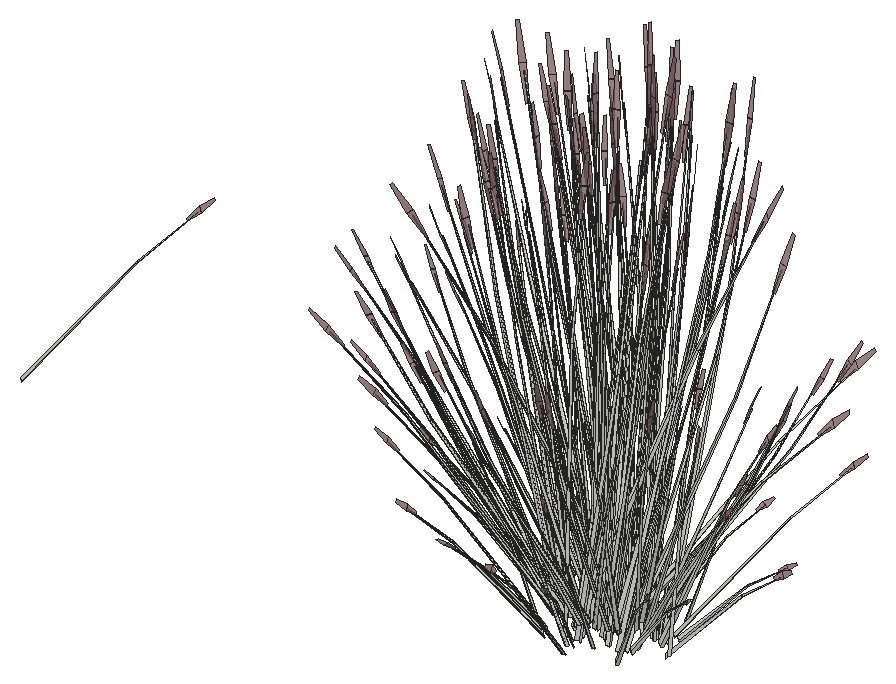
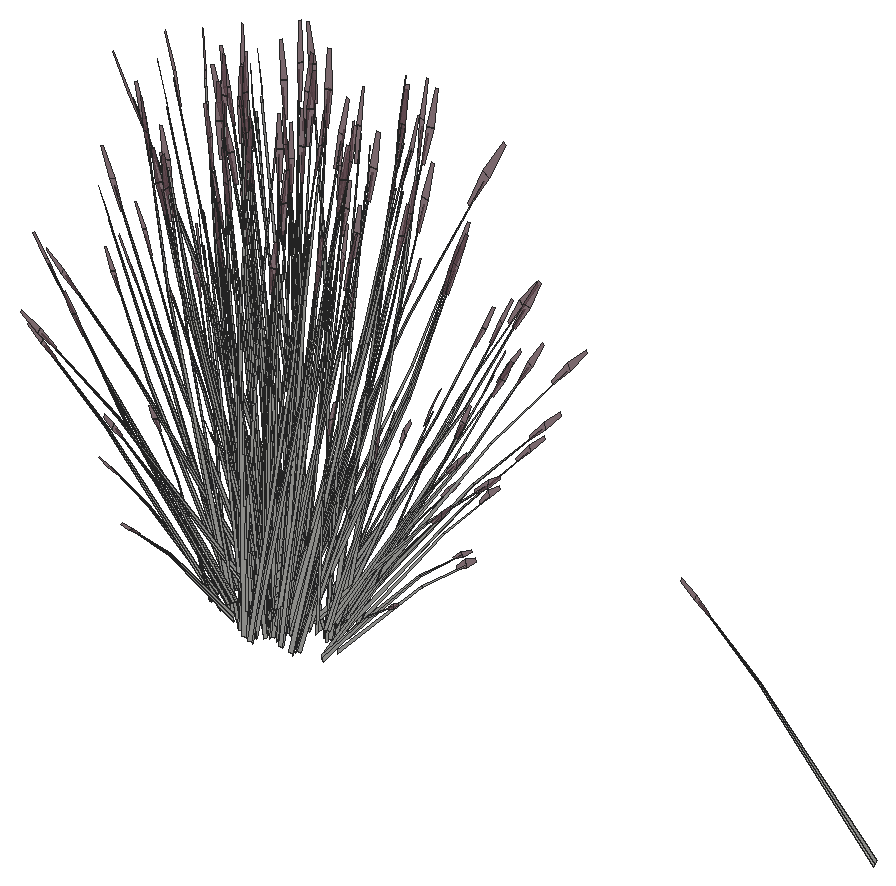
# SketchUp Ruby script. Lengths in millimetres.
U = 1.mm
M = Sketchup.active_model
def pt(a) = Geom::Point3d.new(a.map { |v| v * U })
def face(e, loops, mat)
  f = e.add_face(loops[0].map { |a| pt(a) })
  loops[1..].each { |l| e.add_face(l.map { |a| pt(a) }).erase! }
  f.material = f.back_material = mat if mat
  f
end
# faces: each face lists its corners as indices into pts; further lists are holes
def faces(e, pts, list, mat = nil) = list.each { |f| face(e, (f[0].is_a?(Array) ? f : [f]).map { |l| l.map { |i| pts[i] } }, mat) }
# xy, xz, yz: faces in a plane at the given z, y or x. An outline is a flat list of corners, or four numbers for a rectangle; further outlines are holes
def ring(l) = l.size == 4 ? [[l[0], l[1]], [l[2], l[1]], [l[2], l[3]], [l[0], l[3]]] : l.each_slice(2).to_a
def flat(e, list, mat, &to3) = list.each { |f| face(e, (f[0].is_a?(Array) ? f : [f]).map { |l| ring(l).map { |u, v| to3.(u, v) } }, mat) }
def xy(e, z, list, mat = nil) = flat(e, list, mat) { |x, y| [x, y, z] }
def xz(e, y, list, mat = nil) = flat(e, list, mat) { |x, z| [x, y, z] }
def yz(e, x, list, mat = nil) = flat(e, list, mat) { |y, z| [x, y, z] }
def lines(e, pts, list) = list.each { |a, b| e.add_line(pt(pts[a]), pt(pts[b])) }
# prism: a flat outline (further loops are holes) pulled along v
def prism(e, loops, v, mat = nil)
  f = face(e, loops, mat); d = Geom::Vector3d.new(v.map { |x| x * U })
  f.pushpull(f.normal.samedirection?(d) ? d.length : -d.length)
end
def box(e, o, s, mat = nil) = prism(e, [[o, [o[0] + s[0], o[1], o[2]], [o[0] + s[0], o[1] + s[1], o[2]], [o[0], o[1] + s[1], o[2]]]], [0, 0, s[2]], mat)
def at(x, y, z, deg = 0) = Geom::Transformation.translation(pt([x, y, z])) * Geom::Transformation.rotation(ORIGIN, Z_AXIS, deg.degrees)
def axes(o, x, y, z) = Geom::Transformation.new([*x, 0, *y, 0, *z, 0, *pt(o).to_a, 1])
def part(name) = M.definitions.add(name)
# library, detail: a bought-in or finely detailed component or shape, given as its bounding box
def library(name, o, s) = part(name).tap { |d| box(d.entities, o, s) }
def detail(e, o, s) = box(e.add_group.entities, o, s)
def put(e, d, t, mat = nil) = e.add_instance(d, t).tap { |i| i.material = mat if mat }
def group(e, t, mat = nil) = e.add_group.tap { |g| g.transformation = t; g.material = mat if mat }.entities
root = M.entities
M.materials.add("LightPink_Translucent").color = [144, 107, 117]
M.materials["LightPink_Translucent"].alpha = 0.8
c1 = part("blade")
p = [[54.7,5.3,558.8],[0,4.4,0],[2.3,11.5,0],[55.5,7.8,558.8],[58.2,7.8,558.8],[9.8,11.5,0],
  [62.9,5.7,838.2],[63,6,838.2],[63.4,6,838.2]]
faces(c1.entities,p,[[0,1,2,3],[4,5,2,3],[6,0,3,7],[7,3,4,8]])
c2 = part("seeds")
p = [[7.6,-2.7,35.1],[-0.2,-0.6,40.4],[-0.2,-0.8,0.9],[3.5,-1.8,-1.7],[7.5,-0.8,76.3],[3.7,0.2,78.9]]
faces(c2.entities,p,[[0,1,2,3],[1,0,4,5]],"LightPink_Translucent")
c3 = part("blade with seeds")
put(c3.entities,c1,at(0,0,0))
put(c3.entities,c2,axes([60.9,6.5,787.2],[1.5799,-0.05474,1.17369],[-0.12525,1.92788,0.29478],[-0.07173,-0.02425,1.56792]))
put(root,c3,axes([14344.8,4419.7,8470.3],[-0.29514,-0.25472,1.43002],[0.38401,-0.84262,-0.30754],[0.59714,0.11414,0.61141]))
put(root,c3,axes([16061.4,4330.2,8503],[0.50831,-0.02346,1.71376],[-0.33721,1.01661,0.13857],[-0.72439,-0.06288,0.73262]))
put(root,c3,axes([16066.8,4375.7,8503],[0.42521,-0.21906,1.71376],[0.35798,1.01226,0.13857],[-0.66754,0.22878,0.73262]))
put(root,c3,axes([16033.2,4419.5,8470.3],[0.42589,0.08502,1.43002],[0.2745,0.86839,-0.30754],[-0.57851,0.16255,0.61141]))
put(root,c3,axes([16128.9,4348.8,8489.4],[0.34834,-0.14982,1.77064],[0.12012,1.04605,0.13857],[-0.75452,0.1388,0.63284]))
put(root,c3,axes([16100.1,4306.2,8531],[-1.22504,-0.02494,-0.71045],[0.08228,-1.05005,0.08574],[-0.51899,-0.11081,1.00501]))
put(root,c3,axes([16075,4312.7,8470.3],[0.23927,0.28834,1.43002],[-0.55135,0.78376,-0.30754],[-0.56612,-0.18733,0.61141]))
put(root,c3,axes([16050.1,4352.4,8519.5],[-1.01846,-0.28891,-0.35414],[0.29705,-0.84289,0.4572],[-0.41005,0.07729,0.87481]))
put(root,c3,axes([16085.8,4288.8,8503],[0.45521,0.17844,1.71376],[-0.94204,0.74856,0.13857],[-0.58713,-0.33769,0.73262]))
put(root,c3,axes([16067.8,4363.3,8523.4],[-0.332,0.94205,-0.51099],[-1.13828,-0.3229,-0.3958],[-0.45829,0.08638,0.97773]))
put(root,c3,axes([16089.7,4311.6,8523.4],[-0.88986,0.68603,-0.51099],[-0.77932,-0.72471,-0.3958],[-0.45212,-0.10438,0.97773]))
put(root,c3,axes([16053.3,4361.8,8442.4],[0.03108,0.16322,1.76342],[-0.62654,0.85237,-0.26939],[-0.44504,-0.04296,0.30037]))
put(root,c3,axes([16010.6,4465.7,8474.7],[0.51072,-0.46938,1.1486],[0.20153,0.74307,0.84392],[-0.36908,0.13305,0.25299]))
put(root,c3,axes([16081.3,4295.2,8519.5],[-0.69728,-0.64842,-0.35414],[0.79619,-0.61382,0.4572],[-0.40453,-0.09339,0.87481]))
put(root,c3,axes([16106.3,4393,8503],[0.30609,-0.31822,1.71376],[0.77286,0.85893,0.13857],[-0.53009,0.39116,0.73262]))
put(root,c3,axes([16059.5,4414.1,8519.5],[-1.06674,0.14801,-0.35414],[-0.28168,-0.84611,0.4572],[-0.30569,0.22726,0.87481]))
put(root,c3,axes([16038.8,4334.7,8474.7],[0.78239,-0.07411,1.1486],[-0.49629,0.65296,0.84392],[-0.38663,-0.09795,0.25299]))
put(root,c3,axes([16081.9,4416.7,8523.4],[0.31482,0.94565,-0.51099],[-1.19224,0.16542,-0.3958],[-0.34166,0.254,0.97773]))
put(root,c3,axes([16157.4,4399.4,8456.8],[-1.27479,-0.1698,-0.62353],[0.26901,-1.04736,-0.16365],[-0.38043,-0.12691,1.37633]))
put(root,c3,axes([16154.2,4274.8,8531],[-1.04497,-0.50058,-0.71045],[0.74264,-0.8772,0.08574],[-0.3786,-0.29889,1.00501]))
put(root,c3,axes([16141.7,4275.4,8523.4],[-1.20928,0.24619,-0.51099],[-0.21154,-0.93233,-0.3958],[-0.32481,-0.26718,0.97773]))
put(root,c3,axes([16114.9,4449.8,8455.8],[-1.14694,-0.51783,-0.49651],[0.68554,-0.92854,0],[-0.26122,-0.11794,1.57504]))
put(root,c3,axes([16102.1,4253.9,8442.4],[-0.11871,0.13643,1.76342],[-1.19964,0.29415,-0.26939],[-0.2898,-0.26759,0.30037]))
put(root,c3,axes([16132.6,4465.6,8464.8],[-0.7662,1.03778,0],[-1.28187,-0.57875,-0.51607],[-0.29196,-0.13181,1.63711]))
put(root,c3,axes([16083.2,4267.2,8458.6],[-0.35352,0.84566,-0.03893],[-1.08806,-0.26014,-0.17649],[-0.1652,-0.13832,0.58215]))
put(root,c3,axes([16124.5,4240.1,8470.3],[-0.07421,0.33879,1.43002],[-1.08488,0.28361,-0.30754],[-0.25359,-0.4379,0.61141]))
put(root,c3,axes([16133.5,4262.4,8503],[0.28013,0.33252,1.71376],[-1.29445,0.27994,0.13857],[-0.29256,-0.52202,0.73262]))
put(root,c3,axes([16194.1,4403.4,8472.2],[-1.23732,0.68758,-0.29095],[-0.8228,-0.97154,-0.50002],[-0.30528,-0.09867,1.59708]))
put(root,c3,axes([16145,4258,8519.5],[-0.18927,-0.83419,-0.35414],[1.08199,-0.22027,0.4572],[-0.29062,-0.23905,0.87481]))
put(root,c3,axes([16068.3,4365.3,8464.8],[-1.53239,0,0],[0,-1.1575,-0.51607],[0,-0.26363,1.63711]))
put(root,c3,axes([16123,4440,8456],[-0.28787,-0.90242,-0.30978],[1.14332,-0.25625,0.30978],[-0.23049,-0.10406,1.38974]))
put(root,c3,axes([16215,4422.4,8456.8],[-0.82544,0.77843,-0.62353],[-1.0254,-0.70586,-0.16365],[-0.33076,0.19418,1.37633]))
put(root,c3,axes([16098.5,4357.5,8463.7],[-1.1399,0.87071,0.30756],[-1.1406,-0.86155,-0.36492],[-0.03981,-0.24727,1.64885]))
put(root,c3,axes([16217.7,4418.6,8489],[1.05902,0.41762,1.51261],[-1.03748,0.89969,0.59816],[-0.46471,-0.53324,1.26806]))
put(root,c3,axes([16115,4226.3,8474.7],[0.63926,0.36046,1.1486],[-0.93099,0.21668,0.84392],[-0.1992,-0.27702,0.25299]))
put(root,c3,axes([16229.4,4411.3,8467.1],[-1.19666,-0.83357,-0.25192],[1.00694,-0.93603,0.5513],[-0.32224,0.09751,1.68216]))
put(root,c3,axes([16174.2,4391,8460.7],[-0.73619,-0.86927,-0.44739],[1.11511,-0.61213,0.21531],[-0.23824,-0.10756,1.43643]))
put(root,c3,axes([16214,4406.8,8460.7],[-1.33077,0.06393,-0.44739],[-0.12035,-1.06125,0.21531],[-0.23824,0.10756,1.43643]))
put(root,c3,axes([16149.4,4451.9,8467.5],[1.14694,0.51783,0.49651],[-0.68554,0.92854,0],[-0.26122,-0.11794,1.57504]))
put(root,c3,axes([16176.9,4403.6,8466.5],[0.32481,-1.2272,-0.23429],[1.54007,0.21392,0.51271],[-0.26911,-0.16947,1.5644]))
put(root,c3,axes([16191.1,4411,8471],[-0.23642,0.92427,0.1448],[-1.15506,-0.16044,-0.41347],[-0.21021,-0.09491,1.26744]))
put(root,c3,axes([16249.5,4476.4,8455.8],[-1.14694,0.51783,-0.49651],[-0.68554,-0.92854,0],[-0.26122,0.11794,1.57504]))
put(root,c3,axes([16077,4345.3,8455.8],[0,-1.03566,-0.49651],[1.37109,0,0],[0,-0.23588,1.57504]))
put(root,c3,axes([16092,4369.7,8467.5],[0,1.03566,0.49651],[-1.37109,0,0],[0,-0.23588,1.57504]))
put(root,c3,axes([16251.5,4469.3,8460.2],[-0.75665,-1.04141,-0.05142],[1.28187,-0.57875,0.51607],[-0.31588,0.09915,1.6363]))
put(root,c3,axes([16242.7,4466,8456],[-1.14332,-0.25625,-0.30978],[0.28787,-0.90242,0.30978],[-0.23049,0.10406,1.38974]))
put(root,c3,axes([16168.1,4375.7,8472.2],[-1.38012,-0.49416,-0.29095],[0.66454,-1.04299,-0.50002],[-0.04337,-0.25608,1.59708]))
put(root,c3,axes([16237.7,4399.5,8472.2],[0.1428,1.18174,-0.29095],[-1.48733,0.07145,-0.50002],[-0.26191,0.15741,1.59708]))
put(root,c3,axes([16152.4,4349.1,8457.8],[-0.50328,-1.06202,-0.69835],[1.44974,-0.38248,-0.18329],[-0.05563,-0.35963,1.54149]))
put(root,c3,axes([16209.9,4264.4,8523.4],[-1.20468,-0.25962,-0.51099],[0.41292,-0.89013,-0.3958],[-0.11046,-0.35838,0.97773]))
put(root,c3,axes([16092,4345.9,8456],[0.85545,-0.64616,-0.30978],[0.85545,0.64616,0.30978],[0,-0.20813,1.38974]))
put(root,c3,axes([16190.1,4239.8,8458.6],[-0.84686,0.59414,-0.03893],[-0.77596,-0.65071,-0.17649],[-0.05463,-0.18438,0.58215]))
put(root,c3,axes([16181.4,4388.6,8464.5],[1.54892,0.2182,0.45755],[-0.31522,1.23236,0.17955],[-0.22636,-0.119,1.58856]))
put(root,c3,axes([16171.3,4382.9,8473.6],[-0.59459,0.93321,0.44739],[-1.23546,-0.44912,-0.21531],[0,-0.21512,1.43643]))
put(root,c3,axes([16221.1,4268.7,8531],[-0.5849,-0.8421,-0.71045],[1.20401,-0.4693,0.08574],[-0.13677,-0.40688,1.00501]))
put(root,c3,axes([16160.3,4438.6,8467.4],[1.31687,-0.27488,0.17642],[0.32517,1.02297,0.35086],[-0.11745,-0.14905,1.60407]))
put(root,c3,axes([16203.4,4442.7,8460.3],[-1.23546,-0.46496,0],[0.59459,-0.96613,0],[0,0,1.62707]))
put(root,c3,axes([16259.9,4440,8467.4],[0.35402,-1.02926,0.17642],[1.29548,0.29127,0.35086],[-0.22379,0.00501,1.60407]))
put(root,c3,axes([16244.7,4405.3,8471],[0.90538,0.62224,0.1448],[-0.75521,0.70202,-0.41347],[-0.21021,0.09491,1.26744]))
put(root,c3,axes([16236.5,4385.8,8462.9],[-1.1399,-0.8914,-0.06131],[1.1406,-0.89194,0],[-0.03981,-0.03113,1.75571]))
put(root,c3,axes([16244.1,4393.8,8473.6],[1.33077,-0.06393,0.44739],[0.12035,1.06125,-0.21531],[-0.23824,0.10756,1.43643]))
put(root,c3,axes([16252.3,4455.7,8463.7],[1.53422,0.33662,0.30756],[-0.38383,1.20322,-0.36492],[-0.25393,0.15059,1.64885]))
put(root,c3,axes([16195.5,4221.3,8442.4],[-0.20555,0.03731,1.76342],[-1.13672,-0.42002,-0.26939],[0.01907,-0.35034,0.30037]))
put(root,c3,axes([16269.1,4454,8467.5],[1.14694,-0.51783,0.49651],[0.68554,0.92854,0],[-0.26122,0.11794,1.57504]))
put(root,c3,axes([16223.9,4250.6,8519.5],[0.36946,-0.79643,-0.35414],[1.07787,0.23229,0.4572],[-0.09883,-0.32066,0.87481]))
put(root,c3,axes([16178.1,4359.8,8464.5],[0.53281,1.15808,0.45755],[-1.52239,0.4027,0.17955],[0.01861,-0.2128,1.58856]))
put(root,c3,axes([16171.8,4356,8460.7],[0.59459,-0.93321,-0.44739],[1.23546,0.44912,0.21531],[0,-0.21512,1.43643]))
put(root,c3,axes([16210.5,4432.5,8460.5],[-0.39985,-0.89288,0],[1.1418,-0.31268,0],[0,0,1.54371]))
put(root,c3,axes([16251.5,4387.8,8460.7],[-0.59459,0.93321,-0.44739],[-1.23546,-0.44912,0.21531],[0,0.21512,1.43643]))
put(root,c3,axes([16311.2,4373.3,8467.4],[-0.96285,-0.75439,0.17642],[0.97031,-0.7317,0.35086],[-0.10634,0.15406,1.60407]))
put(root,c3,axes([16226.7,4362.3,8460.5],[0,-1.19833,0],[1.53239,0,0],[0,0,1.79456]))
put(root,c3,axes([16190.5,4367.8,8466.3],[1.3808,0.50196,0.24065],[-0.66454,1.04299,0.50002],[0,-0.24043,1.60543]))
put(root,c3,axes([16246.3,4374.4,8462.7],[0,1.19774,-0.05637],[-1.53239,0,0],[0,0.03764,1.79368]))
put(root,c3,axes([16179.2,4350.1,8473.6],[-1.33077,0.06393,0.44739],[-0.12035,-1.06125,-0.21531],[0.23824,-0.10756,1.43643]))
put(root,c3,axes([16163.5,4303.8,8467.4],[-0.35402,1.02926,0.17642],[-1.29548,-0.29127,0.35086],[0.22379,-0.00501,1.60407]))
put(root,c3,axes([16227.7,4433.3,8462.7],[0.53281,1.18979,-0.06012],[-1.52239,0.41691,0],[0.01861,0.04155,1.72173]))
put(root,c3,axes([16147.4,4271.5,8464.8],[-0.7662,-1.03778,0],[1.28187,-0.57875,-0.51607],[0.29196,-0.13181,1.63711]))
put(root,c3,axes([16339.4,4393.7,8460.4],[-1.53164,-0.00828,-0.04976],[0,-1.1575,0.49943],[-0.04813,0.2635,1.58352]))
put(root,c3,axes([16263,4305.2,8467.4],[-1.31687,0.27488,0.17642],[-0.32517,-1.02297,0.35086],[0.11745,0.14905,1.60407]))
put(root,c3,axes([16228.9,4207.8,8474.7],[0.15721,0.60392,1.1486],[-0.87211,-0.33448,0.84392],[0.09385,-0.30923,0.25299]))
put(root,c3,axes([16208.3,4343.1,8464.5],[-1.01611,0.93987,0.45755],[-1.20717,-0.82966,0.17955],[0.24496,-0.0938,1.58856]))
put(root,c3,axes([16252.4,4380.7,8460.8],[0.85545,0.66896,0],[-0.85545,0.66896,0],[0,0,1.69266]))
put(root,c3,axes([16252.1,4360.9,8473.6],[0.59459,-0.93321,0.44739],[1.23546,0.44912,-0.21531],[0,0.21512,1.43643]))
put(root,c3,axes([16239,4443.2,8460.5],[1.23546,0.46496,0],[-0.59459,0.96613,0],[0,0,1.74954]))
put(root,c3,axes([16241.9,4355.2,8465],[-1.54892,-0.2182,0.49198],[0.31522,-1.23236,0.19306],[0.22636,0.119,1.70813]))
put(root,c3,axes([16331.4,4397.9,8456],[-0.85545,0.64616,-0.30978],[-0.85545,-0.64616,0.30978],[0,0.20813,1.38974]))
put(root,c3,axes([16253.1,4369.1,8460.5],[1.37109,0,0],[0,1.07219,0],[0,0,1.78407]))
put(root,c3,axes([16219.6,4339,8473.6],[-0.73619,-0.86927,0.44739],[1.11511,-0.61213,-0.21531],[0.23824,0.10756,1.43643]))
put(root,c3,axes([16185.6,4344.3,8472.2],[-0.1428,-1.18174,-0.29095],[1.48733,-0.07145,-0.50002],[0.26191,-0.15741,1.59708]))
put(root,c3,axes([16265.2,4366.3,8471],[1.1418,-0.30203,0.1448],[0.39985,0.86246,-0.41347],[0,0.18981,1.26744]))
put(root,c3,axes([16276,4281.6,8523.4],[-0.87728,-0.69587,-0.51099],[0.92674,-0.60943,-0.3958],[0.13348,-0.35356,0.97773]))
put(root,c3,axes([16255.3,4368.1,8472.2],[1.38012,0.49416,-0.29095],[-0.66454,1.04299,-0.50002],[0.04337,0.25608,1.59708]))
put(root,c3,axes([16180.6,4277.8,8456],[1.14332,0.25625,-0.30978],[-0.28787,0.90242,0.30978],[0.23049,-0.10406,1.38974]))
put(root,c3,axes([16261.4,4250.2,8470.3],[-0.34835,0.20963,1.43002],[-1.04325,-0.36691,-0.30754],[0.19338,-0.4563,0.61141]))
put(root,c3,axes([16331.4,4374.1,8467.5],[0,-1.03566,0.49651],[1.37109,0,0],[0,0.23588,1.57504]))
put(root,c3,axes([16346.3,4398.5,8455.8],[0,1.03566,-0.49651],[-1.37109,0,0],[0,0.23588,1.57504]))
put(root,c3,axes([16173.8,4267.4,8455.8],[1.14694,-0.51783,-0.49651],[0.68554,0.92854,0],[0.26122,-0.11794,1.57504]))
put(root,c3,axes([16232.2,4332.8,8471],[0.23642,-0.92427,0.1448],[1.15506,0.16044,-0.41347],[0.21021,0.09491,1.26744]))
put(root,c3,axes([16273.9,4291.9,8467.5],[-1.14694,-0.51783,0.49651],[0.68554,-0.92854,0],[0.26122,0.11794,1.57504]))
put(root,c3,axes([16283,4289.7,8531],[0.03189,-0.95798,-0.71045],[1.34277,0.06434,0.08574],[0.14171,-0.40585,1.00501]))
put(root,c3,axes([16248.5,4429.3,8460],[1.2866,-0.3514,-0.19198],[0.45209,1.01223,0.00008],[0.14202,-0.03884,1.73897]))
put(root,c3,axes([16249.1,4352.9,8460.7],[0.73619,0.86927,-0.44739],[-1.11511,0.61213,0.21531],[0.23824,0.10756,1.43643]))
put(root,c3,axes([16297,4275,8519.5],[0.82919,-0.54528,-0.35414],[0.78493,0.62262,0.4572],[0.11943,-0.31634,0.87481]))
put(root,c3,axes([16302.1,4453.1,8474.7],[-0.69001,-0.29779,1.1486],[0.89096,-0.30257,0.84392],[0.24031,0.2563,0.25299]))
put(root,c3,axes([16208.3,4321.4,8456.8],[0.82544,-0.77843,-0.62353],[1.0254,0.70586,-0.16365],[0.33076,-0.19418,1.37633]))
put(root,c3,axes([16300.3,4303.9,8456],[0.28787,0.90242,-0.30978],[-1.14332,0.25625,0.30978],[0.23049,0.10406,1.38974]))
put(root,c3,axes([16355,4378.6,8464.9],[1.53239,0,0],[0,1.1575,-0.51607],[0,0.26363,1.63711]))
put(root,c3,axes([16229.2,4340.5,8472.2],[1.23732,-0.68758,-0.29095],[0.8228,0.97154,-0.50002],[0.30528,0.09867,1.59708]))
put(root,c3,axes([16244.6,4277.3,8503],[-0.22818,0.35597,1.71376],[-0.95725,-0.73667,0.13857],[0.43183,-0.45914,0.73262]))
put(root,c3,axes([16149.9,4324.9,8445],[-1.20625,0.41464,1.28929],[-0.38394,-1.1897,0.50096],[0.74071,0.01979,1.46642]))
put(root,c3,axes([16290.7,4278.2,8464.9],[0.7662,-1.03778,0],[1.28187,0.57875,-0.51607],[0.29196,0.13181,1.63711]))
put(root,c3,axes([16323.3,4266.6,8442.4],[-0.18342,-0.08159,1.76342],[-0.47115,-0.9115,-0.26939],[0.31784,-0.24736,0.30037]))
put(root,c3,axes([16308.4,4294,8455.8],[1.14694,0.51783,-0.49651],[-0.68554,0.92854,0],[0.26122,0.11794,1.57504]))
put(root,c3,axes([16322.3,4322.3,8523.4],[-0.31482,-0.94565,-0.51099],[1.19224,-0.16542,-0.3958],[0.34166,-0.254,0.97773]))
put(root,c3,axes([16375.6,4446.2,8504.3],[-0.23455,-0.87059,-0.03492],[1.10861,-0.20015,-0.15832],[0.23151,0.05519,0.52218]))
put(root,c3,axes([16265.9,4344.4,8456.8],[1.27479,0.1698,-0.62353],[-0.26901,1.04736,-0.16365],[0.38043,0.12691,1.37633]))
put(root,c3,axes([16403.8,4360.1,8461.9],[-0.75977,-0.66224,-0.06488],[0.83212,-0.6068,-0.29416],[0.23578,-0.04272,0.97024]))
put(root,c3,axes([16359.5,4274.5,8474.7],[-0.40819,0.5272,1.1486],[-0.35086,-0.70831,0.84392],[0.33713,-0.17749,0.25299]))
put(root,c3,axes([16259.2,4401.5,8503],[-0.45521,-0.17844,1.71376],[0.94204,-0.74856,0.13857],[0.58713,0.33769,0.73262]))
put(root,c3,axes([16344.7,4324.8,8519.5],[1.06674,-0.14801,-0.35414],[0.28168,0.84611,0.4572],[0.30569,-0.22726,0.87481]))
put(root,c3,axes([16323.1,4332,8531],[0.64013,-0.81717,-0.71045],[1.12174,0.58074,0.08574],[0.38221,-0.29607,1.00501]))
put(root,c3,axes([16322.9,4443.7,8519.5],[0.69728,0.64842,-0.35414],[-0.79619,0.61382,0.4572],[0.40453,0.09339,0.87481]))
put(root,c3,axes([16336.4,4375.6,8523.4],[0.332,-0.94205,-0.51099],[1.13828,0.3229,-0.3958],[0.45829,-0.08638,0.97773]))
put(root,c3,axes([16409,4390.9,8474.7],[-0.75718,0.17097,1.1486],[0.35641,-0.70661,0.84392],[0.40168,0.04835,0.25299]))
put(root,c3,axes([16346.7,4312.9,8470.3],[-0.4378,-0.03068,1.43002],[-0.44851,-0.8229,-0.30754],[0.53783,-0.23279,0.61141]))
put(root,c3,axes([16354.1,4386.5,8519.5],[1.01846,0.28891,-0.35414],[-0.29705,0.84289,0.4572],[0.41005,-0.07729,0.87481]))
put(root,c3,axes([16304.2,4432.7,8531],[1.22504,0.02494,-0.71045],[-0.08228,1.05005,0.08574],[0.51899,0.11081,1.00501]))
put(root,c3,axes([16367.3,4382.3,8454.9],[-0.7893,0.12429,1.41583],[-0.12563,-0.9893,0.08104],[0.55282,-0.14974,0.80566]))
put(root,c3,axes([16389.2,4365.9,8442.4],[-0.06405,-0.15723,1.76342],[0.44421,-0.91974,-0.26939],[0.4481,-0.01323,0.30037]))
put(root,c3,axes([16283.6,4360,8503],[-0.50831,0.02346,1.71376],[0.33721,-1.01661,0.13857],[0.72439,0.06288,0.73262]))
put(root,c3,axes([16330.9,4384.3,8531],[1.07686,-0.45739,-0.71045],[0.60013,0.94154,0.08574],[0.52031,-0.10696,1.00501]))
put(root,c3,axes([16373,4419.7,8470.3],[-0.29514,-0.25472,1.43002],[0.38401,-0.84262,-0.30754],[0.59714,0.11414,0.61141]))
